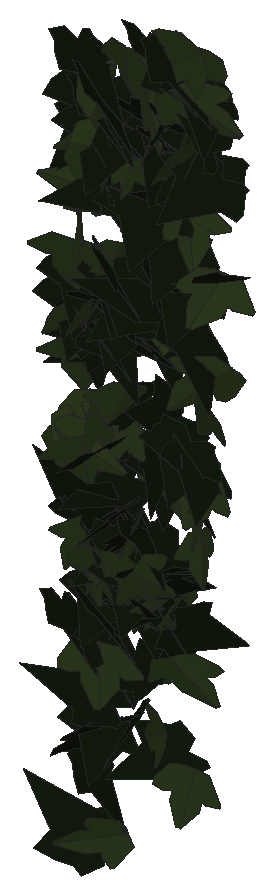
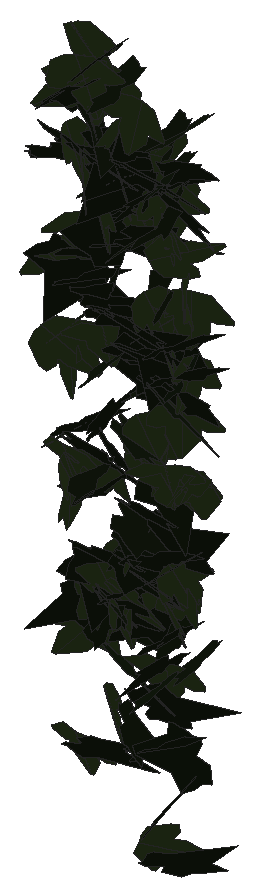
# SketchUp Ruby script. Lengths in inches.
U = 1.inch
M = Sketchup.active_model
def pt(a) = Geom::Point3d.new(a.map { |v| v * U })
def face(e, loops, mat)
  f = e.add_face(loops[0].map { |a| pt(a) })
  loops[1..].each { |l| e.add_face(l.map { |a| pt(a) }).erase! }
  f.material = f.back_material = mat if mat
  f
end
# faces: each face lists its corners as indices into pts; further lists are holes
def faces(e, pts, list, mat = nil) = list.each { |f| face(e, (f[0].is_a?(Array) ? f : [f]).map { |l| l.map { |i| pts[i] } }, mat) }
# xy, xz, yz: faces in a plane at the given z, y or x. An outline is a flat list of corners, or four numbers for a rectangle; further outlines are holes
def ring(l) = l.size == 4 ? [[l[0], l[1]], [l[2], l[1]], [l[2], l[3]], [l[0], l[3]]] : l.each_slice(2).to_a
def flat(e, list, mat, &to3) = list.each { |f| face(e, (f[0].is_a?(Array) ? f : [f]).map { |l| ring(l).map { |u, v| to3.(u, v) } }, mat) }
def xy(e, z, list, mat = nil) = flat(e, list, mat) { |x, y| [x, y, z] }
def xz(e, y, list, mat = nil) = flat(e, list, mat) { |x, z| [x, y, z] }
def yz(e, x, list, mat = nil) = flat(e, list, mat) { |y, z| [x, y, z] }
def lines(e, pts, list) = list.each { |a, b| e.add_line(pt(pts[a]), pt(pts[b])) }
# prism: a flat outline (further loops are holes) pulled along v
def prism(e, loops, v, mat = nil)
  f = face(e, loops, mat); d = Geom::Vector3d.new(v.map { |x| x * U })
  f.pushpull(f.normal.samedirection?(d) ? d.length : -d.length)
end
def box(e, o, s, mat = nil) = prism(e, [[o, [o[0] + s[0], o[1], o[2]], [o[0] + s[0], o[1] + s[1], o[2]], [o[0], o[1] + s[1], o[2]]]], [0, 0, s[2]], mat)
def at(x, y, z, deg = 0) = Geom::Transformation.translation(pt([x, y, z])) * Geom::Transformation.rotation(ORIGIN, Z_AXIS, deg.degrees)
def axes(o, x, y, z) = Geom::Transformation.new([*x, 0, *y, 0, *z, 0, *pt(o).to_a, 1])
def part(name) = M.definitions.add(name)
# library, detail: a bought-in or finely detailed component or shape, given as its bounding box
def library(name, o, s) = part(name).tap { |d| box(d.entities, o, s) }
def detail(e, o, s) = box(e.add_group.entities, o, s)
def put(e, d, t, mat = nil) = e.add_instance(d, t).tap { |i| i.material = mat if mat }
def group(e, t, mat = nil) = e.add_group.tap { |g| g.transformation = t; g.material = mat if mat }.entities
root = M.entities
M.materials.add("1026 AP 7946 SUNNY SIDE UP").color = [254, 231, 186]
M.materials.add("efeu1").color = [18, 25, 13]
M.materials.add("efeu2").color = [43, 57, 29]
c1 = part("ivyleaf_10")
p = [[0,0.5,-0.03],[-0.0625,2.02,-0.43],[-0.19,2.01,-0.46],[-0.54,1.05,-0.29],[-0.52,0.625,-0.18],[-0.83,0.76,-0.28],
  [-1.16,0.64,-0.33],[-1.15,0.33,-0.24],[-0.77,-0.39,0.02],[-0.3,-0.51,0.16],[0.04,-0.48,0.23],[-0.02,2.01,-0.4375],
  [-0.06,2.01,-0.43],[0.04,-0.49,0.23],[0.67,-0.49,0.14],[1.38,0.36,-0.2],[1.375,0.51,-0.24],[0.81,0.65,-0.19],
  [0.62,0.59,-0.15],[0.6,1.09,-0.28],[0.5,1.23,-0.31]]
faces(c1.entities,p,[[0,1,2,3,4,5,6,7,8,9,10],[11,12,0,13,14,15,16,17,18,19,20]],"efeu2")
c2 = part("ivyleaf_9")
p = [[1.54,2.16,1.25],[1.36,2.04,1.19],[-0.21,0.99,0.68],[-0.71,1.11,0.82],[-0.85,0.86,0.67],[-0.8,0.17,0.21],
  [-0.9,-0.01,0.1],[-0.67,-0.16,-0.02],[-0.08,-0.08,-0.05],[-0.03,-0.6,-0.4],[0.65,-0.88,-0.66],[0.83,-0.6,-0.49],
  [1.29,-0.42,-0.43],[1.8125,-0.07,-0.26],[1.21,0.44,0.15]]
faces(c2.entities,p,[[0,1,2,3,4,5,6,7,8,9,10,11,12,13,14]],"efeu1")
put(root,c1,axes([122.42,212.46,276.29],[-0.00767,-0.03696,-0.32932],[-0.12152,0.31026,-0.03395],[0.49085,0.07624,-0.01355]),"1026 AP 7946 SUNNY SIDE UP")
put(root,c1,axes([122.25,212.49,275.22],[-0.10883,-0.25339,-0.14137],[0.10743,0.12117,-0.2681],[0.43908,-0.09245,0.03056]),"1026 AP 7946 SUNNY SIDE UP")
put(root,c2,axes([122.25,212.81,275.24],[-0.2006,-0.2652,0.04179],[0.00799,-0.04895,-0.30232],[0.42214,-0.1251,0.02558]),"1026 AP 7946 SUNNY SIDE UP")
put(root,c2,axes([122.09,212.57,271],[0.16134,-0.26213,0.0003],[-0.00103,-0.00216,-0.29],[0.41218,0.1026,-0.00084]),"1026 AP 7946 SUNNY SIDE UP")
put(root,c2,axes([122.6,212.59,267.83],[-0.38731,-0.21559,-0.02462],[-0.04633,-0.0007,0.33666],[-0.33769,0.24736,-0.01795]),"1026 AP 7946 SUNNY SIDE UP")
put(root,c1,axes([122.35,212.63,274.6],[-0.38121,-0.15554,0.00479],[0.01127,-0.02139,-0.29601],[0.24446,-0.24156,0.02112]),"1026 AP 7946 SUNNY SIDE UP")
put(root,c1,axes([122.38,212.42,276.11],[-0.43943,-0.10349,0.01754],[-0.011,-0.03162,-0.30592],[0.1647,-0.27823,0.02637]),"1026 AP 7946 SUNNY SIDE UP")
put(root,c2,axes([122.59,212.51,272.45],[0.08904,-0.00776,0.28984],[-0.36068,0.1651,0.05321],[-0.25657,-0.23479,0.02579]),"1026 AP 7946 SUNNY SIDE UP")
put(root,c2,axes([122.48,212.79,277.78],[-0.4551,0.0344,-0.09444],[0.13929,-0.03126,-0.29977],[-0.06625,-0.30204,0.01845]),"1026 AP 7946 SUNNY SIDE UP")
put(root,c1,axes([122.55,212.71,276.83],[0.07342,0.12969,0.281],[-0.21515,-0.23615,0.1388],[0.42221,-0.14289,0.02186]),"1026 AP 7946 SUNNY SIDE UP")
put(root,c1,axes([122.45,212.61,272.15],[-0.15933,-0.23349,0.12054],[-0.02309,-0.12162,-0.26089],[0.41095,-0.09736,0.03208]),"1026 AP 7946 SUNNY SIDE UP")
put(root,c2,axes([122.66,212.69,274.82],[-0.35253,0.1892,-0.00598],[-0.01234,-0.01994,-0.30161],[-0.29744,-0.22342,0.0196]),"1026 AP 7946 SUNNY SIDE UP")
put(root,c2,axes([122.35,212.74,275.63],[-0.17117,-0.27678,0.05241],[0.00681,-0.05786,-0.30567],[0.44291,-0.10608,0.02496]),"1026 AP 7946 SUNNY SIDE UP")
put(root,c2,axes([122.31,212.79,274.98],[-0.27778,-0.12224,-0.20391],[0.30431,0.05916,-0.216],[0.20132,-0.25809,0.04514]),"1026 AP 7946 SUNNY SIDE UP")
put(root,c1,axes([122.28,212.64,273.61],[0.27672,0.23068,0.09135],[0.11749,0.05242,-0.29735],[-0.36963,0.18935,-0.02613]),"1026 AP 7946 SUNNY SIDE UP")
put(root,c2,axes([122.25,212.69,278.79],[0.14739,-0.29948,-0.03942],[0.0284,0.04379,-0.32153],[0.47354,0.09059,0.03155]),"1026 AP 7946 SUNNY SIDE UP")
put(root,c1,axes([122.5,212.41,273.4375],[-0.26258,-0.24185,-0.05289],[0.07868,0.02593,-0.30143],[0.38027,-0.17237,0.02585]),"1026 AP 7946 SUNNY SIDE UP")
put(root,c1,axes([122.44,212.81,273.78],[0.3959,0.13956,-0.03498],[-0.0251,-0.04251,-0.29528],[-0.22474,0.25059,-0.02864]),"1026 AP 7946 SUNNY SIDE UP")
put(root,c2,axes([122.39,212.9,272.35],[-0.05701,-0.26367,0.08574],[0.00796,-0.08607,-0.27419],[0.4354,-0.03295,0.01624]),"1026 AP 7946 SUNNY SIDE UP")
put(root,c1,axes([122.45,212.51,271.83],[-0.34491,0.11485,-0.12231],[0.11203,-0.11342,-0.24795],[-0.23516,-0.22249,0.06127]),"1026 AP 7946 SUNNY SIDE UP")
put(root,c1,axes([122.53,212.68,271.7],[0.26386,-0.21763,0.01781],[-0.00393,-0.02527,-0.28269],[0.34342,0.16693,-0.01692]),"1026 AP 7946 SUNNY SIDE UP")
put(root,c1,axes([122.24,212.45,273.45],[-0.20128,-0.0604,-0.26892],[0.41999,-0.04651,-0.12429],[-0.02572,-0.28668,0.07502]),"1026 AP 7946 SUNNY SIDE UP")
put(root,c2,axes([122.4,212.67,268.92],[0.19094,-0.2503,-0.11568],[-0.10608,0.09019,-0.28535],[0.41718,0.1375,-0.01961]),"1026 AP 7946 SUNNY SIDE UP")
put(root,c1,axes([122.6,212.59,275.41],[0.15335,-0.2855,-0.02247],[-0.02386,0.01614,-0.31057],[0.44941,0.09828,-0.00882]),"1026 AP 7946 SUNNY SIDE UP")
put(root,c1,axes([122.61,212.62,277.65],[-0.26002,-0.26247,-0.00736],[0.02284,-0.00247,-0.31929],[0.41217,-0.16544,0.01305]),"1026 AP 7946 SUNNY SIDE UP")
put(root,c2,axes([122.44,212.28,269.36],[-0.00983,0.23091,-0.17711],[-0.00255,0.17324,0.23896],[0.45388,0.00597,-0.00249]),"1026 AP 7946 SUNNY SIDE UP")
put(root,c2,axes([122.54,212.78,271.25],[-0.1315,-0.24277,0.10331],[-0.04433,-0.09779,-0.26504],[0.41146,-0.08812,0.00446]),"1026 AP 7946 SUNNY SIDE UP")
put(root,c2,axes([122.7,212.4375,273.37],[0.00846,0.29668,-0.03841],[-0.00015,-0.03897,-0.30591],[-0.4705,0.00534,-0.00059]),"1026 AP 7946 SUNNY SIDE UP")
put(root,c2,axes([122.42,212.7,277.64],[0.34548,-0.18476,-0.10296],[-0.13345,0.05256,-0.2951],[0.30129,0.23514,-0.01265]),"1026 AP 7946 SUNNY SIDE UP")
put(root,c1,axes([122.61,212.375,275.4],[0.06943,-0.29271,-0.06108],[0.01372,0.05949,-0.3041],[0.4689,0.0416,0.01794]),"1026 AP 7946 SUNNY SIDE UP")
put(root,c2,axes([122.34,212.67,275.14],[0.24599,-0.24185,0.05766],[0.03757,-0.05281,-0.29692],[0.38902,0.15803,-0.00778]),"1026 AP 7946 SUNNY SIDE UP")
put(root,c2,axes([122.52,212.79,278.26],[-0.28223,-0.23408,-0.10237],[0.14155,0.05355,-0.30119],[0.3731,-0.19738,0.03683]),"1026 AP 7946 SUNNY SIDE UP")
put(root,c2,axes([122.96,212.42,269.96],[-0.15024,0.05206,0.27975],[-0.429,0.02695,-0.10417],[-0.06769,-0.28632,0.03932]),"1026 AP 7946 SUNNY SIDE UP")
put(root,c2,axes([122.39,212.76,278.16],[0.19858,-0.28646,-0.01536],[-0.00264,0.01377,-0.32241],[0.4509,0.12624,0.00488]),"1026 AP 7946 SUNNY SIDE UP")
put(root,c1,axes([122.64,212.46,278.16],[0.05777,0.16363,-0.28655],[0.06671,0.27601,0.17409],[0.5043,-0.05526,0.0098]),"1026 AP 7946 SUNNY SIDE UP")
put(root,c2,axes([122.61,212.89,272.5],[-0.24051,-0.2362,-0.01128],[0.04912,-0.00886,-0.28818],[0.36845,-0.153,0.03106]),"1026 AP 7946 SUNNY SIDE UP")
put(root,c1,axes([122.87,212.57,268.04],[0.08528,0.05433,-0.27328],[-0.35283,-0.14297,-0.07817],[-0.23916,0.23029,0.01788]),"1026 AP 7946 SUNNY SIDE UP")
put(root,c2,axes([122.64,212.52,275.47],[0.29621,0.23536,-0.05174],[-0.02309,-0.05411,-0.31005],[-0.37815,0.18766,-0.0216]),"1026 AP 7946 SUNNY SIDE UP")
put(root,c1,axes([122.59,212.65,277.29],[0.29507,-0.2035,0.1251],[0.16538,-0.06891,-0.28411],[0.33495,0.21329,0.03008]),"1026 AP 7946 SUNNY SIDE UP")
put(root,c2,axes([123.02,212.73,276.98],[-0.34825,-0.0649,0.2001],[-0.27855,-0.08391,-0.23701],[0.16267,-0.28263,0.02253]),"1026 AP 7946 SUNNY SIDE UP")
put(root,c2,axes([122.55,212.89,270.54],[0.09888,-0.26432,0.02791],[0.00905,-0.02802,-0.28007],[0.41795,0.06314,-0.00054]),"1026 AP 7946 SUNNY SIDE UP")
put(root,c1,axes([122.8,212.7,276.08],[-0.13929,-0.26627,0.10212],[-0.00129,-0.10516,-0.288],[0.44759,-0.08317,0.03095]),"1026 AP 7946 SUNNY SIDE UP")
put(root,c2,axes([122.69,212.65,269.55],[-0.16232,-0.25938,0.04917],[-0.01,-0.05037,-0.2876],[0.41499,-0.10266,0.0123]),"1026 AP 7946 SUNNY SIDE UP")
put(root,c2,axes([122.49,212.53,271.25],[0.24626,-0.21569,0.06121],[0.05616,-0.04901,-0.27489],[0.3478,0.16064,0.00105]),"1026 AP 7946 SUNNY SIDE UP")
put(root,c1,axes([122.61,212.28,277.7],[-0.03174,-0.13349,-0.2928],[0.28053,0.2286,-0.12266],[0.40499,-0.16881,0.06202]),"1026 AP 7946 SUNNY SIDE UP")
put(root,c1,axes([122.71,212.37,273.94],[0.10787,-0.22024,-0.19367],[0.123,0.19893,-0.21093],[0.43705,-0.00163,0.10716]),"1026 AP 7946 SUNNY SIDE UP")
put(root,c2,axes([123.02,212.72,273],[-0.44244,0.02726,0.02044],[-0.03624,-0.03557,-0.28886],[-0.03849,-0.27981,0.03703]),"1026 AP 7946 SUNNY SIDE UP")
put(root,c2,axes([122.63,212.6,270.82],[0.15314,-0.17968,-0.18932],[-0.05144,0.18519,-0.20445],[0.39969,0.09267,0.04623]),"1026 AP 7946 SUNNY SIDE UP")
put(root,c1,axes([122.84,212.67,277.16],[0.46001,-0.05945,-0.07176],[-0.09987,0.0347,-0.30659],[0.10318,0.29864,0.02318]),"1026 AP 7946 SUNNY SIDE UP")
put(root,c1,axes([122.86,212.7,273.68],[0.42482,-0.07944,-0.07798],[-0.11859,0.01004,-0.28982],[0.12466,0.28027,-0.00995]),"1026 AP 7946 SUNNY SIDE UP")
put(root,c2,axes([122.82,212.625,277.89],[-0.29266,-0.24951,-0.00584],[0.02126,-0.00479,-0.3204],[0.39182,-0.18611,0.01303]),"1026 AP 7946 SUNNY SIDE UP")
put(root,c1,axes([122.83,212.43,271.93],[-0.44353,-0.04352,-0.03305],[0.05612,-0.02363,-0.29268],[0.06355,-0.28287,0.02783]),"1026 AP 7946 SUNNY SIDE UP")
put(root,c2,axes([122.64,212.7,277.79],[0.15339,-0.23037,-0.17991],[-0.00878,0.18144,-0.2506],[0.45323,0.08148,0.05604]),"1026 AP 7946 SUNNY SIDE UP")
put(root,c2,axes([122.6,212.53,278.44],[0.21689,-0.26749,0.08071],[0.03344,-0.07876,-0.31003],[0.43767,0.13857,-0.01631]),"1026 AP 7946 SUNNY SIDE UP")
put(root,c2,axes([123.15,212.79,278],[-0.47677,0.04882,0.04663],[-0.08412,-0.05511,-0.31014],[-0.06182,-0.30154,0.06236]),"1026 AP 7946 SUNNY SIDE UP")
put(root,c1,axes([122.75,212.41,270.58],[0.46847,0.05719,0.04297],[0.07098,-0.01634,-0.31162],[-0.08534,0.30035,-0.02331]),"1026 AP 7946 SUNNY SIDE UP")
put(root,c2,axes([122.66,212.7,274.93],[0.04685,-0.29435,-0.00339],[0.0781,0.00663,-0.30035],[0.45621,0.02909,0.05176]),"1026 AP 7946 SUNNY SIDE UP")
put(root,c2,axes([123.0625,212.73,272.01],[-0.4289,0.04061,-0.02436],[0.02541,-0.0511,-0.28007],[-0.06958,-0.269,0.04785]),"1026 AP 7946 SUNNY SIDE UP")
put(root,c1,axes([122.96,212.66,274.19],[-0.17482,-0.25006,0.09067],[-0.02902,-0.08944,-0.28181],[0.41658,-0.11117,0.01842]),"1026 AP 7946 SUNNY SIDE UP")
put(root,c2,axes([122.77,212.77,275.7],[-0.07177,-0.27318,0.11597],[0.01246,-0.11656,-0.28485],[0.46536,-0.03901,0.02551]),"1026 AP 7946 SUNNY SIDE UP")
put(root,c2,axes([122.93,212.79,275.36],[-0.36238,-0.17273,-0.08206],[0.13031,0.01976,-0.29467],[0.2685,-0.24272,0.03226]),"1026 AP 7946 SUNNY SIDE UP")
put(root,c2,axes([123.12,212.79,272.83],[-0.28702,0.1545,-0.154],[0.06821,-0.16668,-0.23165],[-0.33207,-0.16778,0.08553]),"1026 AP 7946 SUNNY SIDE UP")
put(root,c2,axes([123.08,212.74,272.28],[-0.14774,0.1758,-0.19993],[0.06464,-0.19477,-0.20237],[-0.40781,-0.09456,0.04035]),"1026 AP 7946 SUNNY SIDE UP")
put(root,c2,axes([123.18,212.72,274.1],[-0.32006,0.2024,-0.05403],[0.00347,-0.07268,-0.29178],[-0.32921,-0.19754,0.04946]),"1026 AP 7946 SUNNY SIDE UP")
put(root,c2,axes([123.11,212.68,272.67],[-0.21127,0.16502,-0.19135],[0.06812,-0.19338,-0.20937],[-0.38581,-0.12451,0.06781]),"1026 AP 7946 SUNNY SIDE UP")
put(root,c2,axes([123.26,212.7,275.29],[0.04347,0.04636,0.30561],[-0.42668,0.13078,0.00577],[-0.20113,-0.26741,0.05381]),"1026 AP 7946 SUNNY SIDE UP")
put(root,c2,axes([122.8,212.41,276.16],[0.35521,-0.20063,-0.07953],[-0.11737,0.03006,-0.3099],[0.3163,0.23646,-0.02568]),"1026 AP 7946 SUNNY SIDE UP")
put(root,c1,axes([123.02,212.72,278.84],[-0.45541,0.0951,-0.01115],[-0.00078,-0.03768,-0.31207],[-0.1506,-0.28739,0.03533]),"1026 AP 7946 SUNNY SIDE UP")
put(root,c1,axes([123.3,212.77,271.69],[-0.20829,0.10535,0.22415],[-0.37885,-0.06951,-0.11717],[0.01795,-0.24453,0.12806]),"1026 AP 7946 SUNNY SIDE UP")
put(root,c2,axes([123.2,212.86,275.76],[-0.46449,0.00409,-0.01234],[0.01812,-0.02985,-0.30299],[-0.0083,-0.29413,0.02884]),"1026 AP 7946 SUNNY SIDE UP")
put(root,c2,axes([122.63,212.65,275.09],[0.27848,-0.11876,0.22551],[0.26194,-0.14428,-0.21966],[0.29234,0.24241,-0.01799]),"1026 AP 7946 SUNNY SIDE UP")
put(root,c1,axes([123.08,212.8,272.32],[-0.05622,0.09776,-0.26529],[-0.04075,-0.26027,-0.0994],[-0.43202,0.01183,0.0439]),"1026 AP 7946 SUNNY SIDE UP")
put(root,c2,axes([122.92,212.82,277.05],[0.13954,-0.29033,-0.02999],[-0.00096,0.02852,-0.31249],[0.45855,0.08841,0.00847]),"1026 AP 7946 SUNNY SIDE UP")
put(root,c2,axes([123.14,212.77,269.8],[-0.2267,0.03559,-0.23885],[0.26219,-0.17618,-0.13559],[-0.25986,-0.2088,0.07157]),"1026 AP 7946 SUNNY SIDE UP")
put(root,c1,axes([123.11,212.58,277.56],[0.38689,-0.17101,0.04164],[0.03301,-0.04211,-0.30808],[0.27469,0.24593,-0.02162]),"1026 AP 7946 SUNNY SIDE UP")
put(root,c2,axes([122.93,212.5,271.44],[0.44806,-0.03445,0.00293],[-0.00045,-0.02761,-0.2945],[0.05438,0.28363,-0.02661]),"1026 AP 7946 SUNNY SIDE UP")
put(root,c2,axes([123.13,212.72,271.72],[-0.17858,-0.25944,0.03847],[0.00013,-0.04233,-0.29149],[0.41248,-0.11231,0.01675]),"1026 AP 7946 SUNNY SIDE UP")
put(root,c1,axes([123.29,212.6875,271.47],[-0.03254,-0.27519,0.01376],[-0.00204,-0.01486,-0.28438],[0.43334,-0.02073,-0.0003]),"1026 AP 7946 SUNNY SIDE UP")
put(root,c2,axes([123.53,212.54,270.61],[-0.34454,0.18742,0.02162],[-0.04604,-0.00367,-0.29622],[-0.29276,-0.21999,0.02114]),"1026 AP 7946 SUNNY SIDE UP")
put(root,c2,axes([123.1,212.68,278.2],[0.478,0.0291,-0.03712],[-0.05255,-0.02935,-0.31365],[-0.05071,0.30473,-0.02485]),"1026 AP 7946 SUNNY SIDE UP")
put(root,c1,axes([123.3,212.72,277.85],[0.20906,-0.27901,0.00541],[0.03064,0.00173,-0.31783],[0.43777,0.13312,0.01966]),"1026 AP 7946 SUNNY SIDE UP")
put(root,c2,axes([123.48,212.59,275.69],[-0.42315,-0.10159,0.05368],[-0.05301,-0.05827,-0.29351],[0.17196,-0.26796,0.04161]),"1026 AP 7946 SUNNY SIDE UP")
put(root,c2,axes([123.1,212.71,272.4],[0.1476,-0.25273,0.05995],[0.02222,-0.05834,-0.27799],[0.4077,0.09468,-0.00656]),"1026 AP 7946 SUNNY SIDE UP")
put(root,c2,axes([123.4375,212.74,275.91],[-0.3998,-0.15132,-0.01028],[0.03061,-0.01493,-0.304],[0.23639,-0.25398,0.02198]),"1026 AP 7946 SUNNY SIDE UP")
put(root,c2,axes([123.19,212.69,277.85],[0.4722,0.00767,-0.05554],[-0.08458,-0.00703,-0.30946],[-0.01382,0.30504,-0.00395]),"1026 AP 7946 SUNNY SIDE UP")
put(root,c1,axes([123.56,212.76,271.84],[-0.38979,-0.05658,0.12744],[-0.17029,-0.07459,-0.25848],[0.13019,-0.26696,0.04346]),"1026 AP 7946 SUNNY SIDE UP")
put(root,c2,axes([123.29,212.76,271.54],[-0.29334,-0.11826,-0.18381],[0.26458,0.06385,-0.22532],[0.20663,-0.24964,0.02756]),"1026 AP 7946 SUNNY SIDE UP")
put(root,c2,axes([123.78,212.58,275.65],[-0.22471,0.02777,0.2921],[-0.44771,-0.01137,-0.14684],[-0.00363,-0.31717,0.02897]),"1026 AP 7946 SUNNY SIDE UP")
put(root,c2,axes([123.57,212.66,271.56],[-0.3535,0.13299,-0.09435],[0.0936,-0.07905,-0.26705],[-0.23675,-0.22983,0.0353]),"1026 AP 7946 SUNNY SIDE UP")
put(root,c1,axes([123.39,212.62,271.45],[-0.33888,0.16547,-0.05234],[0.04172,-0.0501,-0.27919],[-0.2694,-0.21591,0.0226]),"1026 AP 7946 SUNNY SIDE UP")
put(root,c2,axes([123.7,212.9,269.35],[-0.39465,-0.06957,0.10936],[-0.15145,-0.05011,-0.26774],[0.13076,-0.26802,0.01995]),"1026 AP 7946 SUNNY SIDE UP")
put(root,c1,axes([123.43,212.59,278.45],[-0.04482,0.30566,-0.00994],[-0.02217,-0.01274,-0.31594],[-0.48045,-0.02792,0.0155]),"1026 AP 7946 SUNNY SIDE UP")
put(root,c2,axes([123.59,212.58,271.95],[0.17491,0.21017,-0.14674],[-0.10414,-0.12746,-0.24572],[-0.38649,0.12946,-0.0002]),"1026 AP 7946 SUNNY SIDE UP")
put(root,c2,axes([123.4,212.91,273.27],[-0.06524,-0.27622,0.05309],[-0.00436,-0.05328,-0.28802],[0.44226,-0.04127,0.00499]),"1026 AP 7946 SUNNY SIDE UP")
put(root,c2,axes([123.5,212.58,277.07],[-0.33021,-0.21394,-0.04186],[0.07382,0.00893,-0.30753],[0.33401,-0.21349,0.02658]),"1026 AP 7946 SUNNY SIDE UP")
put(root,c2,axes([123.62,212.83,272.21],[-0.42203,-0.06562,-0.03477],[0.06775,-0.03769,-0.28081],[0.09387,-0.26783,0.04635]),"1026 AP 7946 SUNNY SIDE UP")
put(root,c2,axes([123.26,212.68,276.77],[0.51541,0.05577,0.00917],[-0.02216,0.03194,0.34094],[0.08591,-0.32633,0.03295]),"1026 AP 7946 SUNNY SIDE UP")
put(root,c2,axes([123.36,212.89,275.0625],[0.07224,-0.28299,0.06052],[0.00833,-0.06027,-0.29567],[0.45491,0.04604,-0.0042]),"1026 AP 7946 SUNNY SIDE UP")
put(root,c1,axes([123.48,212.8125,275.47],[0.40357,0.1431,-0.03205],[-0.02455,-0.03732,-0.30186],[-0.22923,0.25593,-0.0241]),"1026 AP 7946 SUNNY SIDE UP")
put(root,c2,axes([123.26,212.77,279.12],[0.18043,-0.27576,0.09039],[0.10304,-0.06888,-0.30626],[0.44398,0.12805,0.03435]),"1026 AP 7946 SUNNY SIDE UP")
put(root,c2,axes([123.64,212.77,274],[-0.11086,-0.01779,0.29361],[-0.22415,-0.25228,-0.05401],[0.38924,-0.15035,0.05251]),"1026 AP 7946 SUNNY SIDE UP")
put(root,c1,axes([123.625,212.67,271.45],[-0.22221,-0.24631,0.01972],[0.00086,-0.02397,-0.29241],[0.38865,-0.14078,0.01192]),"1026 AP 7946 SUNNY SIDE UP")
put(root,c1,axes([123.7,212.41,269.84],[0.15863,-0.1475,-0.21742],[-0.14276,0.19078,-0.18168],[0.37771,0.13406,0.02264]),"1026 AP 7946 SUNNY SIDE UP")
put(root,c2,axes([123.72,212.5,278.24],[0.00254,0.22548,0.25448],[0.00594,0.24572,-0.23085],[-0.52438,0.00387,-0.00138]),"1026 AP 7946 SUNNY SIDE UP")
put(root,c1,axes([123.51,212.26,272.03],[-0.12596,-0.19583,-0.22503],[0.17593,0.18769,-0.21561],[0.42501,-0.13573,0.02256]),"1026 AP 7946 SUNNY SIDE UP")
put(root,c2,axes([123.37,212.86,271.19],[0.28614,-0.134,-0.16686],[0.2379,-0.06381,0.23021],[-0.22816,-0.23459,0.03077]),"1026 AP 7946 SUNNY SIDE UP")
put(root,c2,axes([123.51,212.8,277.63],[-0.12519,-0.24181,0.176],[0.00434,-0.17889,-0.25851],[0.46677,-0.06319,0.0496]),"1026 AP 7946 SUNNY SIDE UP")
put(root,c2,axes([123.46,212.66,276.1],[0.16979,-0.24792,-0.14184],[0.25505,-0.06525,0.25433],[-0.36447,-0.16116,0.11189]),"1026 AP 7946 SUNNY SIDE UP")
put(root,c2,axes([123.92,212.81,273.68],[-0.39894,0.09246,0.09171],[-0.14384,0.00642,-0.27704],[-0.14075,-0.26862,0.02319]),"1026 AP 7946 SUNNY SIDE UP")
put(root,c2,axes([123.625,212.57,271.83],[0.24028,0.22717,-0.03976],[-0.01749,-0.04053,-0.28195],[-0.36224,0.15264,-0.01276]),"1026 AP 7946 SUNNY SIDE UP")
put(root,c1,axes([123.64,212.71,277.28],[0.29915,-0.24062,-0.04939],[-0.00054,0.0587,-0.31351],[0.38538,0.18686,0.0379]),"1026 AP 7946 SUNNY SIDE UP")
put(root,c1,axes([123.71,212.76,278.57],[0.17098,-0.29184,-0.03853],[-0.00045,0.03801,-0.32034],[0.46232,0.10797,0.01394]),"1026 AP 7946 SUNNY SIDE UP")
put(root,c2,axes([123.6,212.58,273.71],[-0.2796,-0.02049,-0.23746],[0.35836,-0.06507,-0.17563],[-0.06202,-0.28366,0.05569]),"1026 AP 7946 SUNNY SIDE UP")
put(root,c1,axes([123.61,212.68,273.375],[-0.40974,0.02956,-0.12905],[0.1539,-0.13868,-0.24395],[-0.13182,-0.25378,0.11632]),"1026 AP 7946 SUNNY SIDE UP")
put(root,c1,axes([123.93,212.77,279.18],[-0.43616,-0.08553,0.10649],[-0.13942,-0.06276,-0.2976],[0.15911,-0.28946,0.03114]),"1026 AP 7946 SUNNY SIDE UP")
put(root,c2,axes([123.77,212.77,276.58],[-0.29232,-0.24099,0.02163],[0.04584,-0.05029,-0.30893],[0.37778,-0.18037,0.05422]),"1026 AP 7946 SUNNY SIDE UP")
put(root,c1,axes([123.58,212.46,278.97],[-0.38179,-0.00183,-0.21307],[0.31947,-0.0618,-0.24553],[-0.06087,-0.31291,0.04784]),"1026 AP 7946 SUNNY SIDE UP")
put(root,c2,axes([123.57,212.88,273.3],[0.21006,-0.24669,0.05577],[0.02758,-0.05362,-0.28914],[0.39664,0.13437,-0.00943]),"1026 AP 7946 SUNNY SIDE UP")
put(root,c2,axes([124.24,212.71,277.97],[-0.27319,0.17028,0.19168],[-0.26373,0.08918,-0.2462],[-0.29469,-0.23768,0.04264]),"1026 AP 7946 SUNNY SIDE UP")
put(root,c1,axes([123.88,212.71,277.78],[0.12163,-0.28903,-0.0845],[0.02698,0.08714,-0.30526],[0.47095,0.06965,0.03931]),"1026 AP 7946 SUNNY SIDE UP")
put(root,c1,axes([123.96,212.43,277.95],[0.01898,-0.29787,-0.09796],[0.00869,0.09365,-0.30643],[0.49078,0.00986,0.00921]),"1026 AP 7946 SUNNY SIDE UP")
put(root,c2,axes([123.74,212.55,279.3],[0.15577,-0.28347,-0.10124],[-0.04326,0.09277,-0.30877],[0.46895,0.10272,0.00515]),"1026 AP 7946 SUNNY SIDE UP")
put(root,c2,axes([123.95,212.72,276.06],[-0.20813,-0.26714,0.0439],[-0.00728,-0.04688,-0.30694],[0.42568,-0.13142,0.01621]),"1026 AP 7946 SUNNY SIDE UP")
put(root,c1,axes([124.18,212.37,279.41],[0.33639,-0.11159,-0.21844],[-0.27045,0.12517,-0.24665],[0.26104,0.27348,0.02596]),"1026 AP 7946 SUNNY SIDE UP")
put(root,c2,axes([123.88,212.76,278.92],[-0.09821,-0.30326,-0.04693],[0.03271,0.04044,-0.31849],[0.48068,-0.06471,0.01208]),"1026 AP 7946 SUNNY SIDE UP")
put(root,c1,axes([123.95,212.7,276.95],[0.20495,0.27218,-0.03419],[-0.00604,-0.03664,-0.31085],[-0.4314,0.12982,-0.01189]),"1026 AP 7946 SUNNY SIDE UP")
put(root,c2,axes([123.91,212.56,271.32],[0.09231,0.0083,-0.28752],[-0.07114,0.28175,0.00048],[0.43331,0.04449,0.06133]),"1026 AP 7946 SUNNY SIDE UP")
put(root,c1,axes([124.1,212.69,278.1],[0.02834,-0.31066,-0.00819],[-0.01071,0.0058,-0.32047],[0.48846,0.01815,-0.00655]),"1026 AP 7946 SUNNY SIDE UP")
put(root,c2,axes([124.02,212.61,273.87],[-0.18071,-0.26589,0.07485],[-0.01772,-0.07575,-0.2982],[0.43369,-0.11388,0.01901]),"1026 AP 7946 SUNNY SIDE UP")
put(root,c1,axes([124.01,212.61,269.2],[0.43941,-0.05716,0.02562],[0.03034,-0.03085,-0.29278],[0.09342,0.27888,-0.02542]),"1026 AP 7946 SUNNY SIDE UP")
put(root,c1,axes([123.98,212.46,270.84],[-0.35543,-0.08943,-0.15528],[0.23477,0.02897,-0.24906],[0.14299,-0.26985,0.02296]),"1026 AP 7946 SUNNY SIDE UP")
put(root,c2,axes([124.3,212.8,277.89],[-0.40391,-0.15316,0.06661],[-0.05465,-0.06851,-0.30572],[0.25619,-0.25609,0.03981]),"1026 AP 7946 SUNNY SIDE UP")
put(root,c2,axes([124.12,212.54,276.16],[0.26397,0.24446,0.04991],[0.04734,0.03641,-0.30527],[-0.38858,0.1705,-0.00328]),"1026 AP 7946 SUNNY SIDE UP")
put(root,c2,axes([124,212.67,275.42],[0.04468,-0.33704,0.05917],[0.00557,-0.05926,-0.34879],[0.53808,0.0286,-0.0013]),"1026 AP 7946 SUNNY SIDE UP")
put(root,c2,axes([124.09,212.77,278.82],[-0.05472,-0.30725,0.05374],[-0.00019,-0.05423,-0.31881],[0.4905,-0.03429,0.00587]),"1026 AP 7946 SUNNY SIDE UP")
put(root,c1,axes([124.2,212.62,273.36],[0.43304,-0.08012,-0.0053],[-0.01813,-0.02292,-0.29447],[0.12489,0.27448,-0.02438]),"1026 AP 7946 SUNNY SIDE UP")
put(root,c1,axes([124.45,212.62,274.98],[-0.22412,-0.19067,0.23405],[-0.16871,-0.20312,-0.24499],[0.43618,-0.17654,0.0255]),"1026 AP 7946 SUNNY SIDE UP")
put(root,c2,axes([124.18,212.61,273.69],[-0.06811,-0.27461,0.11031],[0.01299,-0.11088,-0.28601],[0.46417,-0.03719,0.02419]),"1026 AP 7946 SUNNY SIDE UP")
put(root,c1,axes([124.25,212.63,273.13],[0.0774,-0.23597,0.15826],[0.11537,-0.1412,-0.24635],[0.42865,0.08061,0.03772]),"1026 AP 7946 SUNNY SIDE UP")
put(root,c1,axes([124.1,212.42,278.79],[-0.29552,-0.11983,-0.23562],[0.3471,0.07058,-0.22522],[0.20879,-0.28695,0.04093]),"1026 AP 7946 SUNNY SIDE UP")
put(root,c1,axes([124.26,212.49,272.66],[-0.02371,-0.27388,0.05616],[0.1593,-0.05769,-0.26256],[0.40969,0.00658,0.10534]),"1026 AP 7946 SUNNY SIDE UP")
put(root,c1,axes([124.38,212.6875,276.18],[0.32629,0.17052,-0.14023],[-0.14738,-0.10144,-0.27675],[-0.31087,0.22707,-0.01598]),"1026 AP 7946 SUNNY SIDE UP")
put(root,c1,axes([124.53,212.29,274.68],[-0.32371,0.15001,0.17644],[-0.23531,0.08334,-0.26133],[-0.26846,-0.25393,0.01631]),"1026 AP 7946 SUNNY SIDE UP")
put(root,c2,axes([124.48,212.6,277.71],[-0.36438,-0.16844,0.10283],[-0.06902,-0.1075,-0.28972],[0.30082,-0.22869,0.05809]),"1026 AP 7946 SUNNY SIDE UP")
